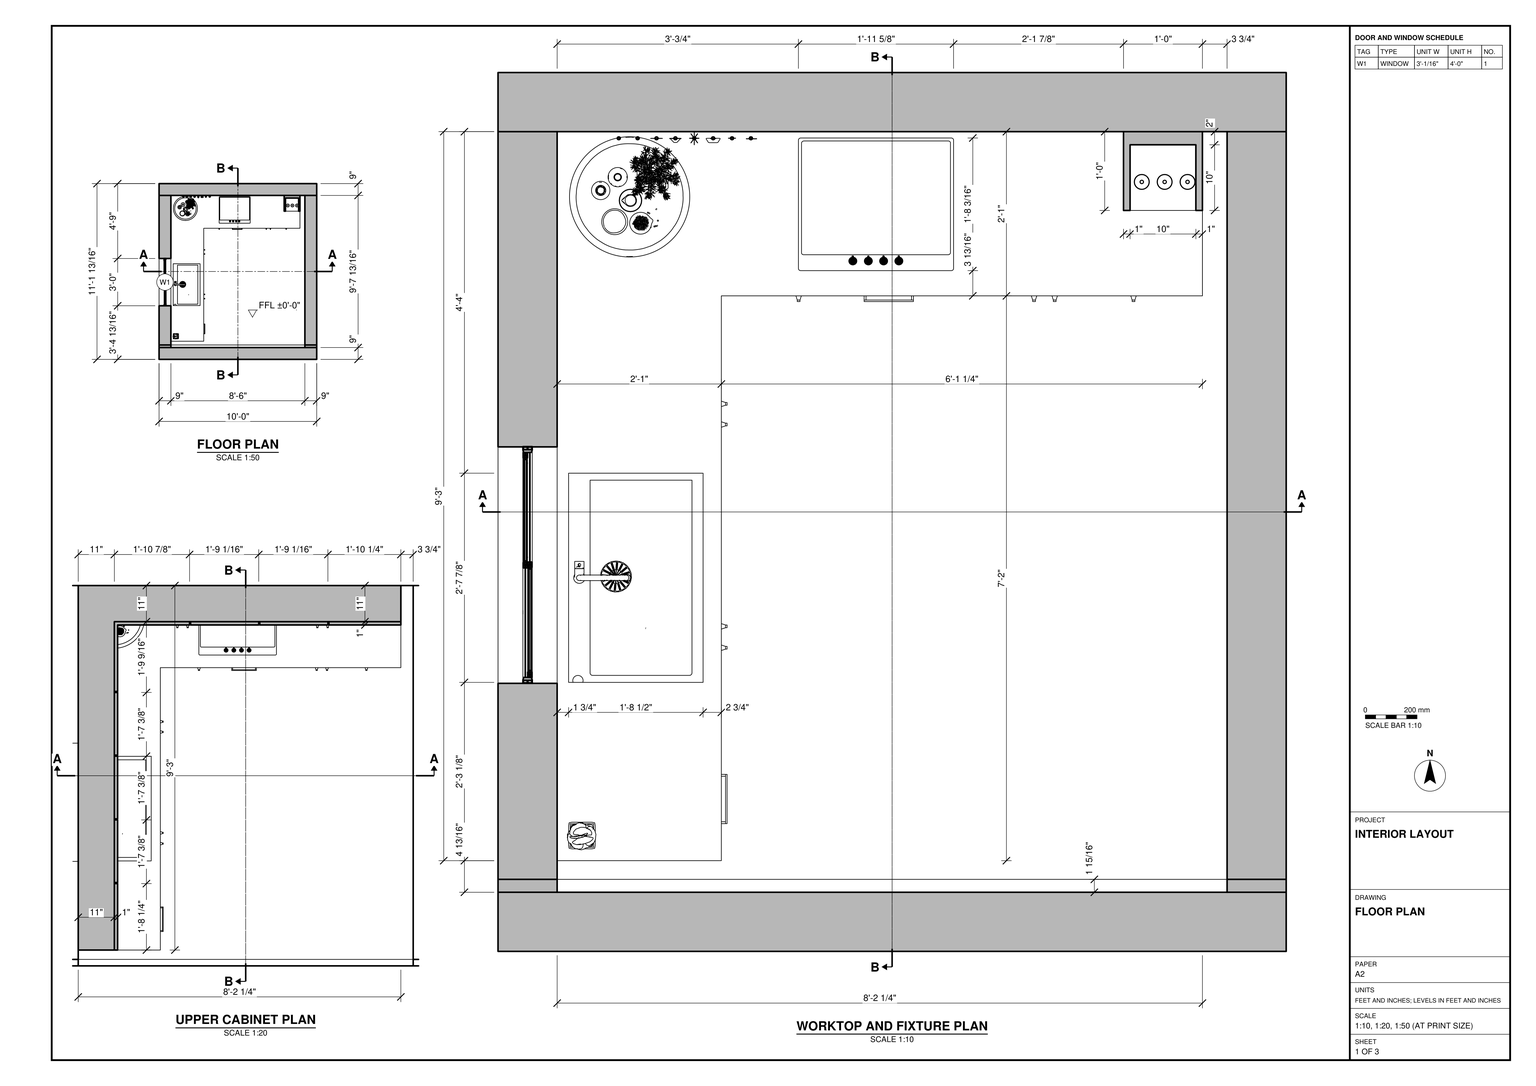
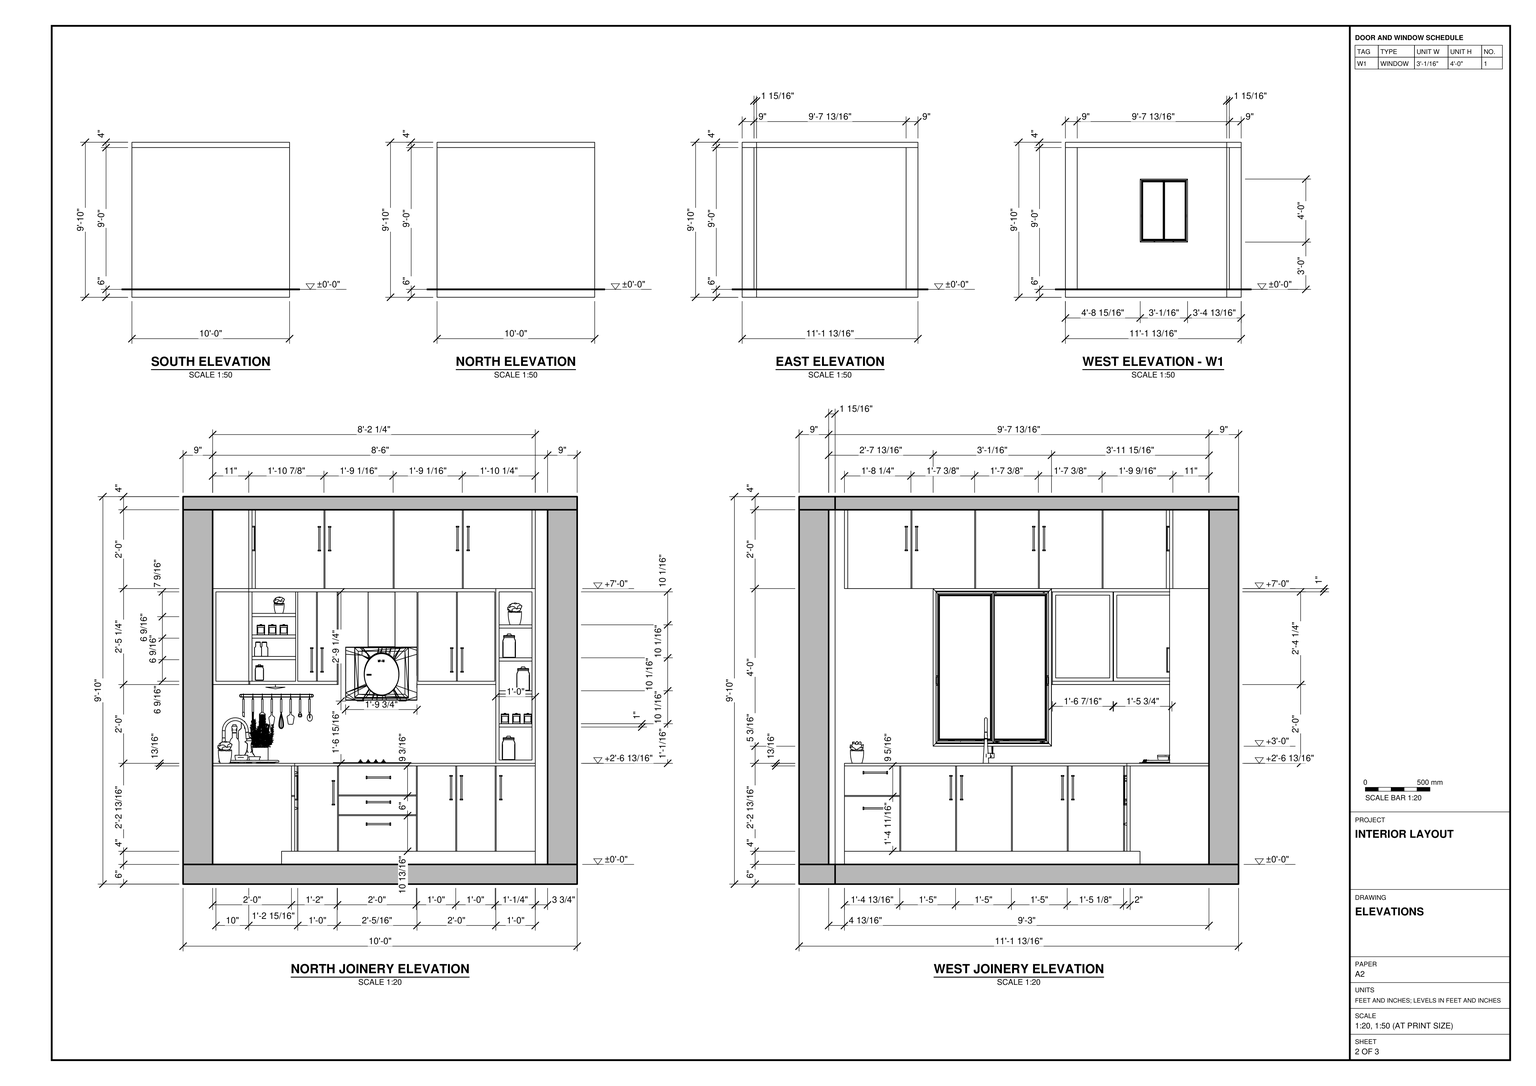
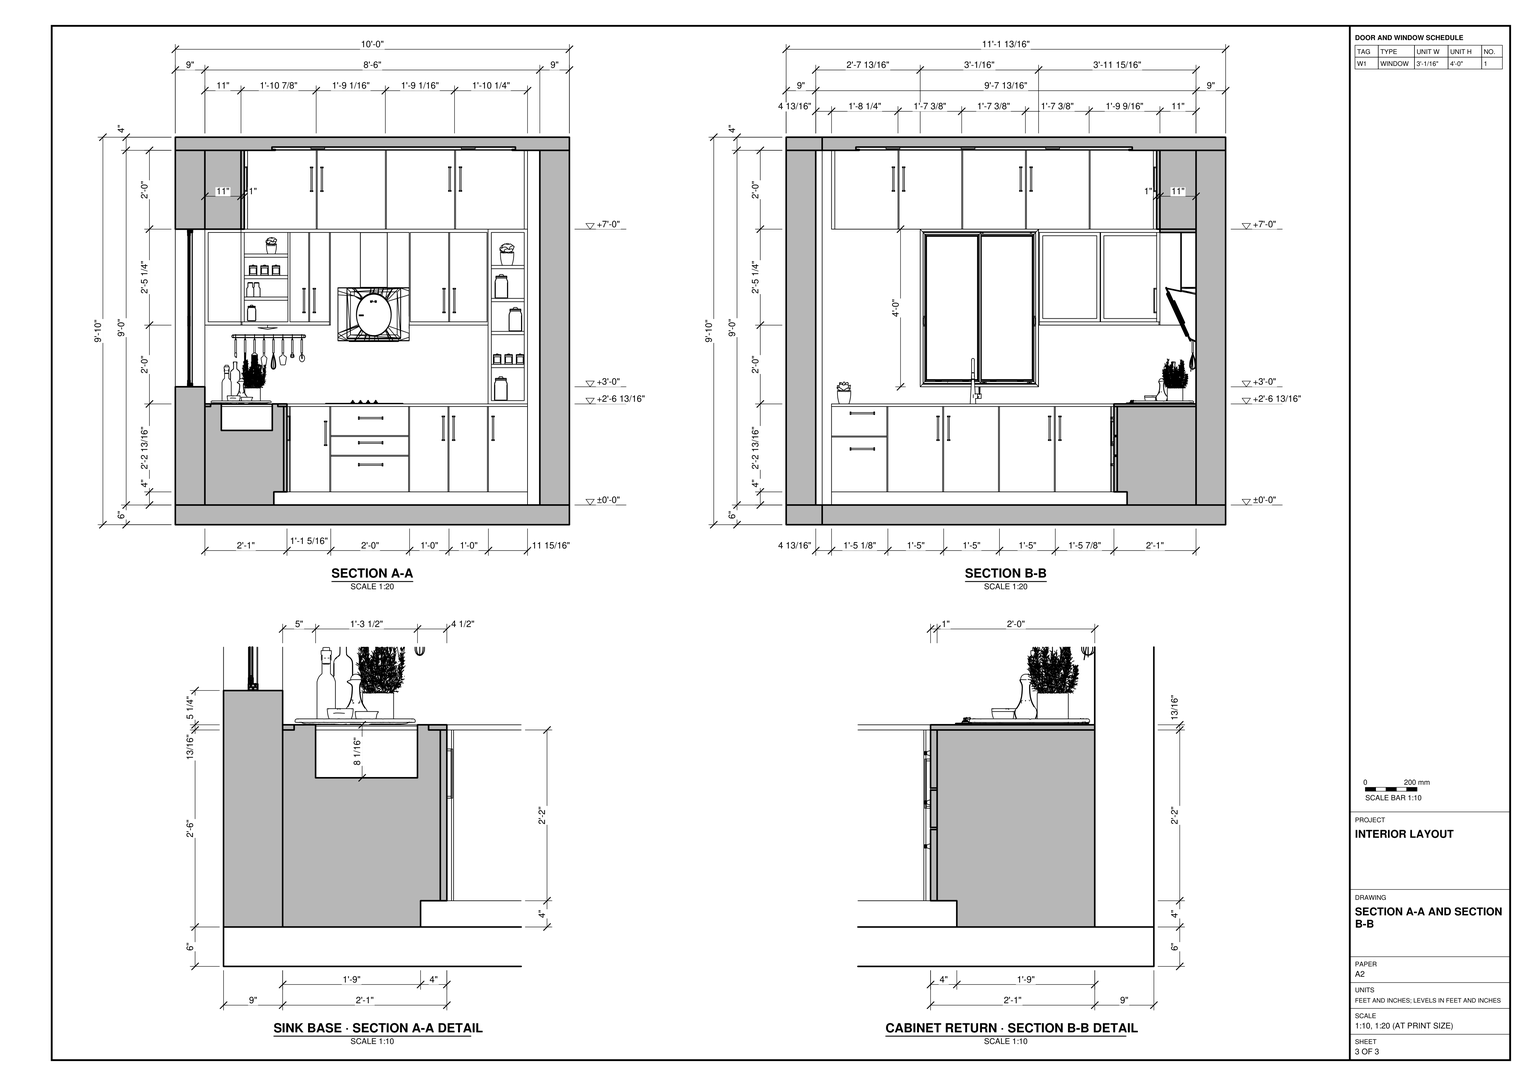
Build the kitchen in SketchUp from task_files/diagram_01.pdf. Work in feet and inches. Set the finished floor at ±0'-0". The room shell measures 10'-0" east to west by 11'-1 13/16" north to south, with an overall height of 9'-10". Model the 9" perimeter walls between the 6" floor slab and the 4" top slab. Fit the two-panel window in the west wall, with its sill above the sink as shown in the section.

Use the worktop plan to lay out the continuous L-shaped counter, with the sink and faucet on the west run and the cooktop on the north run. Follow the joinery elevations for the base cupboards, drawer stacks, handles, open shelves and upper cabinets. Align the extractor hood with the cooktop and the drawers below it. Use the enlarged sections to set the basin into the worktop and recess the plinths behind the cabinet fronts. Keep the upper cabinets clear of the window opening.

Decor, appliances and loose items such as jars, utensils and plants may be any suitable library components placed as shown. Keep shell elements and individual furniture or joinery pieces in separate groups or components, and use components for repeated parts. Save one SketchUp model as output_files/kitchen_with_l_shaped_cabinetry_and_a_west_window.skp.

# SketchUp Ruby script. Lengths in inches.
U = 1.inch
M = Sketchup.active_model
def pt(a) = Geom::Point3d.new(a.map { |v| v * U })
def face(e, loops, mat)
  f = e.add_face(loops[0].map { |a| pt(a) })
  loops[1..].each { |l| e.add_face(l.map { |a| pt(a) }).erase! }
  f.material = f.back_material = mat if mat
  f
end
# faces: each face lists its corners as indices into pts; further lists are holes
def faces(e, pts, list, mat = nil) = list.each { |f| face(e, (f[0].is_a?(Array) ? f : [f]).map { |l| l.map { |i| pts[i] } }, mat) }
# xy, xz, yz: faces in a plane at the given z, y or x. An outline is a flat list of corners, or four numbers for a rectangle; further outlines are holes
def ring(l) = l.size == 4 ? [[l[0], l[1]], [l[2], l[1]], [l[2], l[3]], [l[0], l[3]]] : l.each_slice(2).to_a
def flat(e, list, mat, &to3) = list.each { |f| face(e, (f[0].is_a?(Array) ? f : [f]).map { |l| ring(l).map { |u, v| to3.(u, v) } }, mat) }
def xy(e, z, list, mat = nil) = flat(e, list, mat) { |x, y| [x, y, z] }
def xz(e, y, list, mat = nil) = flat(e, list, mat) { |x, z| [x, y, z] }
def yz(e, x, list, mat = nil) = flat(e, list, mat) { |y, z| [x, y, z] }
def lines(e, pts, list) = list.each { |a, b| e.add_line(pt(pts[a]), pt(pts[b])) }
# prism: a flat outline (further loops are holes) pulled along v
def prism(e, loops, v, mat = nil)
  f = face(e, loops, mat); d = Geom::Vector3d.new(v.map { |x| x * U })
  f.pushpull(f.normal.samedirection?(d) ? d.length : -d.length)
end
def box(e, o, s, mat = nil) = prism(e, [[o, [o[0] + s[0], o[1], o[2]], [o[0] + s[0], o[1] + s[1], o[2]], [o[0], o[1] + s[1], o[2]]]], [0, 0, s[2]], mat)
def at(x, y, z, deg = 0) = Geom::Transformation.translation(pt([x, y, z])) * Geom::Transformation.rotation(ORIGIN, Z_AXIS, deg.degrees)
def axes(o, x, y, z) = Geom::Transformation.new([*x, 0, *y, 0, *z, 0, *pt(o).to_a, 1])
def part(name) = M.definitions.add(name)
# library, detail: a bought-in or finely detailed component or shape, given as its bounding box
def library(name, o, s) = part(name).tap { |d| box(d.entities, o, s) }
def detail(e, o, s) = box(e.add_group.entities, o, s)
def put(e, d, t, mat = nil) = e.add_instance(d, t).tap { |i| i.material = mat if mat }
def group(e, t, mat = nil) = e.add_group.tap { |g| g.transformation = t; g.material = mat if mat }.entities
root = M.entities
M.materials.add("Emissive").color = [255, 242, 225]
M.materials["Emissive"].alpha = 1
M.materials.add("Manhattan Creative Coating ML 1016B 24.75cm").color = [255, 255, 255]
M.materials.add("Marble Beige 23-86 150cm").color = [204, 192, 177]
M.materials.add("Marble Black 01 150cm").color = [31, 31, 31]
M.materials.add("Wood Mahogany 33-46 100cm\#2").color = [84, 42, 21]
M.materials.add("Wood Teak 33-35 100cm").color = [135, 81, 33]
M.materials.add("[Color M09]").color = [0, 0, 0]
M.materials.add("[Translucent Glass Blue]").color = [100, 149, 237]
M.materials["[Translucent Glass Blue]"].alpha = 0.5
c1 = library("Window Crafter Sliding",[0,-0.1,0],[78.74,3.59,94.49])
c2 = part("Square panel")
box(c2.entities,[0,0,0],[10.02,10,1],"Wood Mahogany 33-46 100cm\#2")
c3 = part("Component\#4")
box(c3.entities,[0,1,0],[13.97,9,1])
c4 = part("Component\#6")
box(c4.entities,[0,0,0],[9,18.46,1])
c5 = part("Component\#7")
box(c5.entities,[0,0,0],[9,17.75,1])
c6 = library("sink",[-18.39,0,-10.63],[31.85,20.47,24.5])
c7 = library("Chimney",[0,-14.34,0],[33.95,14.34,33.72])
c8 = part("POI-E1497-320-1917\#1")
xy(c8.entities,0,[[0,0,0.29,0.83],[7.21,0,7.5,0.83]])
xy(c8.entities,0.64,[[0.29,0.21,7.21,0.62]])
xy(c8.entities,0.875,[[0,0.21,7.5,0.62]])
xz(c8.entities,0.21,[[0,0.64,7.5,0.875]])
xz(c8.entities,0.62,[[0,0.64,7.5,0.875]])
yz(c8.entities,0,[[0,0,0.21,0.64,0.21,0.875,0.62,0.875,0.62,0.64,0.83,0]])
yz(c8.entities,0.29,[[0,0,0.83,0,0.62,0.64,0.21,0.64]])
yz(c8.entities,7.21,[[0,0,0.21,0.64,0.62,0.64,0.83,0]])
yz(c8.entities,7.5,[[0,0,0.83,0,0.62,0.64,0.62,0.875,0.21,0.875,0.21,0.64]])
p = [[0,0.21,0.64],[0,0,0],[0.29,0,0],[0.29,0.21,0.64],[7.21,0.21,0.64],[7.21,0,0],
  [7.5,0,0],[7.5,0.21,0.64],[0,0.83,0],[0,0.62,0.64],[0.29,0.62,0.64],[0.29,0.83,0],
  [7.5,0.83,0],[7.5,0.62,0.64],[7.21,0.62,0.64],[7.21,0.83,0]]
faces(c8.entities,p,[[0,1,2,3],[4,5,6,7],[8,9,10,11],[12,13,14,15]])
c9 = library("1045",[78.33,40.52,-0.08],[23.62,20.2,1.2])
c10 = library("kitchen",[57.57,5.21,10.61],[18.31,18.31,13.72])
c11 = library("Kitchen Utensils 20-56",[-15.41,-1.59,-10.72],[30.82,2.02,11.3])
c12 = library("Glass Vessel 001",[-1.95,-1.95,0.02],[3.9,3.9,7.26])
c13 = library("Kitchen Utensils Jugs 92-07",[-4.45,-3.74,0],[8.9,7.5,9.62])
c14 = library("jars",[-1.97,-1.97,0],[15.75,3.94,5.39])
c15 = library("Potted Plant 50-24",[-2.18,-2.1,0],[4.36,4.2,6.7])
c16 = part("Group319\#1")
p = [[0,0,0],[0,0,-1.83],[-0.77,0,-1.83],[5.01,-0.92,0],[-5.01,-0.92,0],[5.01,0.92,0],
  [5.01,0,0],[-5.01,0.92,0],[0.77,0,-1.83],[-5.01,0,0],[0,0,-2.96]]
lines(c16.entities,p,[[0,1],[1,2],[3,4],[5,6],[7,5],[1,8],[9,0],[0,6],[8,10],[4,9],[6,3],[2,10],
  [9,7]])
c17 = part("Rectangle Light")
put(c17.entities,c16,at(0,0,0))
c18 = part("Group321\#1")
p = [[0,0,0],[0,0,-1.81],[-0.77,0,-1.81],[5.01,-0.84,0],[-5.01,-0.84,0],[5.01,0.84,0],
  [5.01,0,0],[-5.01,0.84,0],[0.77,0,-1.81],[-5.01,0,0],[0,0,-2.93]]
lines(c18.entities,p,[[0,1],[1,2],[3,4],[5,6],[7,5],[1,8],[9,0],[0,6],[8,10],[4,9],[6,3],[2,10],
  [9,7]])
c19 = part("Rectangle Light\#1")
put(c19.entities,c18,at(0,0,0))
c20 = part("Group323\#1")
p = [[0,0,0],[0,0,-2],[-0.77,0,-2],[5.01,-1.47,0],[-5.01,-1.47,0],[5.01,1.47,0],
  [5.01,0,0],[-5.01,1.47,0],[0.77,0,-2],[-5.01,0,0],[0,0,-3.24]]
lines(c20.entities,p,[[0,1],[1,2],[3,4],[5,6],[7,5],[1,8],[9,0],[0,6],[8,10],[4,9],[6,3],[2,10],
  [9,7]])
c21 = part("Rectangle Light\#2")
put(c21.entities,c20,at(0,0,0))
c22 = part("Group325\#3")
p = [[0,0,0],[0,0,-1.85],[-0.77,0,-1.85],[5.01,-0.98,0],[-5.01,-0.98,0],[5.01,0.98,0],
  [5.01,0,0],[-5.01,0.98,0],[0.77,0,-1.85],[-5.01,0,0],[0,0,-2.99]]
lines(c22.entities,p,[[0,1],[1,2],[3,4],[5,6],[7,5],[1,8],[9,0],[0,6],[8,10],[4,9],[6,3],[2,10],
  [9,7]])
c23 = part("Rectangle Light\#3")
put(c23.entities,c22,at(0,0,0))
c24 = part("Group327\#1")
p = [[0,0,0],[0,0,-1.97],[-0.77,0,-1.97],[5.01,-1.38,0],[-5.01,-1.38,0],[5.01,1.38,0],
  [5.01,0,0],[-5.01,1.38,0],[0.77,0,-1.97],[-5.01,0,0],[0,0,-3.19]]
lines(c24.entities,p,[[0,1],[1,2],[3,4],[5,6],[7,5],[1,8],[9,0],[0,6],[8,10],[4,9],[6,3],[2,10],
  [9,7]])
c25 = part("Rectangle Light\#4")
put(c25.entities,c24,at(0,0,0))
c26 = part("Group329\#1")
p = [[0,0,0],[0,0,-2.64],[-1.07,0,-2.64],[6.99,-1.58,0],[-6.99,-1.58,0],[6.99,1.58,0],
  [6.99,0,0],[-6.99,1.58,0],[1.07,0,-2.64],[-6.99,0,0],[0,0,-4.28]]
lines(c26.entities,p,[[0,1],[1,2],[3,4],[5,6],[7,5],[1,8],[9,0],[0,6],[8,10],[4,9],[6,3],[2,10],
  [9,7]])
c27 = part("Rectangle Light\#5")
put(c27.entities,c26,at(0,0,0))
c28 = part("Group331\#1")
p = [[0,0,0],[0,0,-2.47],[-1.07,0,-2.47],[6.99,-1.01,0],[-6.99,-1.01,0],[6.99,1.01,0],
  [6.99,0,0],[-6.99,1.01,0],[1.07,0,-2.47],[-6.99,0,0],[0,0,-4]]
lines(c28.entities,p,[[0,1],[1,2],[3,4],[5,6],[7,5],[1,8],[9,0],[0,6],[8,10],[4,9],[6,3],[2,10],
  [9,7]])
c29 = part("Rectangle Light\#6")
put(c29.entities,c28,at(0,0,0))
c30 = part("Group333\#1")
p = [[0,0,0],[0,0,-2.5],[-1.07,0,-2.5],[6.99,-1.09,0],[-6.99,-1.09,0],[6.99,1.09,0],
  [6.99,0,0],[-6.99,1.09,0],[1.07,0,-2.5],[-6.99,0,0],[0,0,-4.04]]
lines(c30.entities,p,[[0,1],[1,2],[3,4],[5,6],[7,5],[1,8],[9,0],[0,6],[8,10],[4,9],[6,3],[2,10],
  [9,7]])
c31 = part("Rectangle Light\#7")
put(c31.entities,c30,at(0,0,0))
c32 = part("Group335\#1")
p = [[0,0,0],[0,0,-2.52],[-1.07,0,-2.52],[6.99,-1.16,0],[-6.99,-1.16,0],[6.99,1.16,0],
  [6.99,0,0],[-6.99,1.16,0],[1.07,0,-2.52],[-6.99,0,0],[0,0,-4.07]]
lines(c32.entities,p,[[0,1],[1,2],[3,4],[5,6],[7,5],[1,8],[9,0],[0,6],[8,10],[4,9],[6,3],[2,10],
  [9,7]])
c33 = part("Rectangle Light\#8")
put(c33.entities,c32,at(0,0,0))
c34 = library("Tlon Light 650 Ceiling 152 007",[-12.8,-12.8,-3.78],[25.6,25.6,3.58])
c35 = part("Group347\#3")
p = [[0,0,0],[0,0,-4.23],[-1.84,0,-4.23],[12,-1.68,0],[-12,-1.68,0],[12,1.68,0],
  [12,0,0],[-12,1.68,0],[1.84,0,-4.23],[-12,0,0],[0,0,-6.84]]
lines(c35.entities,p,[[0,1],[1,2],[3,4],[5,6],[7,5],[1,8],[9,0],[0,6],[8,10],[4,9],[6,3],[2,10],
  [9,7]])
c36 = part("Rectangle Light\#10")
put(c36.entities,c35,at(0,0,0))
c37 = library("Group\#23",[-0.04,-0.04,0],[3.03,9.65,3.68])
c38 = part("Group345\#1")
p = [[0,0,0],[0,0,-6.68],[-2.9375,0,-6.68],[19.12,-2.51,0],[-19.12,-2.51,0],[19.12,2.51,0],
  [19.12,0,0],[-19.12,2.51,0],[2.9375,0,-6.68],[-19.12,0,0],[0,0,-10.8125]]
lines(c38.entities,p,[[0,1],[1,2],[3,4],[5,6],[7,5],[1,8],[9,0],[0,6],[8,10],[4,9],[6,3],[2,10],
  [9,7]])
c39 = part("Rectangle Light\#9")
put(c39.entities,c38,at(0,0,0))
c40 = part("Group343\#1")
xz(c40.entities,22.6,[[26.53,0,146.53,6]])
c41 = part("Group347\#1")
xz(c41.entities,22.6,[[26.53,6,35.53,114]])
c42 = part("Group1235\#1")
xz(c42.entities,22.6,[[137.53,6,146.53,114]])
c43 = part("Group1237\#1")
xz(c43.entities,22.6,[[26.53,114,146.53,118]])
c44 = part("Group340\#3")
put(c44.entities,c40,at(0,0,0))
put(c44.entities,c41,at(0,0,0))
put(c44.entities,c42,at(0,0,0))
put(c44.entities,c43,at(0,0,0))
box(root,[0,0,6],[120,9,108])
p = [[71.02,100.8125,10],[47.34,100.8125,10],[71.02,100.8125,20.84],[71.02,100.8125,26.84],[47.34,100.8125,26.84],[47.34,100.8125,21.16],
  [71.02,100.8125,21.16],[47.34,100.8125,20.84],[29.1875,42.02,36],[29.24,42.03,36],[29.29,42.05,36],[29.33,42.07,36],
  [14.26,42.05,36],[14.31,42.03,36],[14.07,42.22,36],[14.1,42.17,36],[29.5,42.26,36],[29.52,42.3125,36],
  [14.03,42.3125,36],[14.04,42.26,36],[14.02,42.42,36],[14.02,42.36,36],[14.17,42.1,36],[14.21,42.07,36],
  [14.13,42.13,36],[14.36,42.02,36],[14.41,42.02,36],[29.53,71.75,36],[14.02,71.75,36],[29.13,42.02,36],
  [29.41,42.13,36],[29.45,42.17,36],[29.375,42.1,36],[29.48,42.22,36],[29.52,42.36,36],[12.16,56.0625,36.79],
  [12.38,56.03,36.79],[11.95,56.15,36.79],[11.76,56.28,36.79],[11.625,56.46,36.79],[11.54,56.66,36.79],[11.51,56.88,36.79],
  [11.54,57.1,36.79],[11.625,57.3,36.79],[11.76,57.48,36.79],[11.95,57.61,36.79],[12.16,57.7,36.79],[12.38,57.73,36.79],
  [12.61,57.7,36.79],[12.82,57.61,36.79],[13,57.48,36.79],[13.14,57.3,36.79],[13.22,57.1,36.79],[13.25,56.88,36.79],
  [13.22,56.66,36.79],[13.14,56.46,36.79],[13,56.28,36.79],[12.82,56.15,36.79],[12.61,56.0625,36.79],[33,47.65,10],
  [33,47.65,36],[71.02,100.8125,27.16],[71.02,100.8125,36],[33,100.8125,10],[47.02,100.8125,10],[107.25,100.8125,10],
  [107.25,100.8125,36],[95.02,100.8125,10],[83.34,100.8125,10],[33,100.8125,36],[33,64.64,10],[33,64.96,10],
  [33,47.96,10],[95.34,100.8125,10],[33,30.97,36],[33,30.97,10],[33,13.8125,27],[33,13.8125,36],
  [95.02,100.8125,36],[47.34,100.8125,27.16],[71.34,100.8125,36],[71.34,100.8125,10],[83.02,100.8125,10],[83.02,100.8125,36],
  [33,81.64,10],[33,81.64,36],[33,30.65,27],[83.34,100.8125,36],[95.23,124.8125,36.79],[95.23,112.8125,36.79],
  [107.25,112.8125,36.79],[33,13.8125,26.69],[33,13.8125,10],[33,81.95,10],[33,81.95,36],[33,30.65,26.69],
  [33,30.65,10],[47.02,100.8125,36],[33,64.64,36],[33,30.65,36],[33,47.96,36],[33,64.96,36],
  [47.34,100.8125,36],[107.25,124.8125,36.79],[95.34,100.8125,36],[107.25,124.8125,6],[107.25,103.8125,6],[9,124.8125,6],
  [9,13.8125,6],[30,13.8125,6],[30,103.8125,6],[9,13.8125,36],[9,13.8125,36.79],[9,124.8125,36],
  [107.25,124.8125,36],[9,124.8125,36.79]]
lines(root,p,[[0,1],[0,2],[3,4],[4,5],[5,6],[2,7],[7,1],[6,3],[8,9],[10,11],[12,13],[14,15],
  [16,17],[18,19],[20,21],[22,23],[24,22],[13,25],[25,26],[27,28],[26,29],[23,12],[9,10],[30,31],
  [21,18],[11,32],[31,33],[15,24],[33,16],[32,30],[19,14],[29,8],[17,34],[34,27],[28,20],[35,36],
  [37,35],[38,37],[39,38],[40,39],[41,40],[42,41],[43,42],[44,43],[45,44],[46,45],[47,46],[48,47],
  [49,48],[50,49],[51,50],[52,51],[53,52],[54,53],[55,54],[56,55],[57,56],[58,57],[36,58],[59,60],
  [61,62],[63,64],[65,66],[67,68],[69,63],[70,71],[59,72],[65,73],[74,75],[76,77],[67,78],[79,61],
  [80,81],[72,70],[82,83],[84,85],[76,86],[75,59],[87,68],[88,89],[89,90],[91,92],[84,93],[94,93],
  [95,91],[92,96],[64,97],[70,98],[96,95],[71,84],[86,99],[100,72],[101,71],[102,79],[90,103],[96,75],
  [93,63],[82,81],[104,73],[105,106],[105,107],[107,108],[109,110],[106,110],[74,60],[77,99],[111,77],[111,112],
  [113,111],[114,66],[114,103],[114,113],[103,88],[113,115],[69,97],[108,111],[107,113],[105,114],[115,112],[100,98],
  [85,94],[104,66],[78,104],[80,83],[97,102],[88,115],[101,85],[87,78],[62,80],[60,100],[62,102],[99,74],
  [83,87],[94,69],[98,101],[109,108]])
put(root,c1,axes([3.79,76.86,42],[0,-0.4578,0],[0.42,0,0],[0,0,0.508]))
put(root,c2,at(96.23,112.8125,47.83))
put(root,c2,at(96.23,112.8125,57.87))
put(root,c2,at(96.23,112.8125,67.91))
put(root,c2,at(96.23,112.8125,77.96),"Wood Mahogany 33-46 100cm\#2")
put(root,c3,at(20.31,113.8125,68.34))
put(root,c3,at(20.31,113.8125,74.89))
put(root,c3,at(20.31,113.8125,81.45))
put(root,c4,at(10,77.13,70.52))
put(root,c4,at(10,77.13,79.26))
put(root,c5,at(10,95.75,70.52))
put(root,c5,at(10,95.75,79.26))
put(root,c6,at(31.22,59.34,36.79,90))
put(root,c7,axes([49.5,124.8125,54.79],[0.64,0,0],[0,0.64,0],[0,0,1.01456]))
put(root,c8,axes([34,26.95,34.36],[0,-1,0],[0,0,-1],[1,0,0]))
put(root,c8,axes([34,26.95,23.48],[0,-1,0],[0,0,-1],[1,0,0]))
put(root,c8,axes([63.24,99.8125,32.88],[-1,0,0],[0,0,-1],[0,-1,0]))
put(root,c8,axes([34,45.82,33.11],[0,0,-1],[0,1,0],[1,0,0]))
put(root,c8,axes([34,79.81,33.11],[0,0,-1],[0,1,0],[1,0,0]))
put(root,c8,axes([34,49.08,33.11],[0,0,-1],[0,1,0],[1,0,0]))
put(root,c8,axes([34,82.95,33.11],[0,0,-1],[0,1,0],[1,0,0]))
put(root,c8,axes([63.24,99.8125,25.38],[-1,0,0],[0,0,-1],[0,-1,0]))
put(root,c8,axes([63.24,99.8125,18.69],[-1,0,0],[0,0,-1],[0,-1,0]))
put(root,c8,axes([45.35,99.8125,31.57],[0,0,-1],[1,0,0],[0,-1,0]))
put(root,c8,axes([96.34,99.8125,33.11],[0,0,-1],[1,0,0],[0,-1,0]))
put(root,c8,axes([84.34,99.8125,33.11],[0,0,-1],[1,0,0],[0,-1,0]))
put(root,c8,axes([81.19,99.8125,33.11],[0,0,-1],[1,0,0],[0,-1,0]))
put(root,c8,axes([41.07,112.8125,108.9375],[0,0,-1],[1,0,0],[0,-1,0]))
put(root,c8,axes([44.22,112.8125,108.9375],[0,0,-1],[1,0,0],[0,-1,0]))
put(root,c8,axes([86.41,112.8125,109],[0,0,-1],[1,0,0],[0,-1,0]))
put(root,c8,axes([83.16,112.8125,109],[0,0,-1],[1,0,0],[0,-1,0]))
put(root,c8,axes([21,32.23,109],[0,0,-1],[0,1,0],[1,0,0]))
put(root,c8,axes([21,71.03,109],[0,0,-1],[0,1,0],[1,0,0]))
put(root,c8,axes([21,74.17,109],[0,0,-1],[0,1,0],[1,0,0]))
put(root,c8,axes([21,35.37,109],[0,0,-1],[0,1,0],[1,0,0]))
put(root,c9,at(-32.59,63.125,36.87))
put(root,c10,at(-46.6875,100.52,26.18))
put(root,c11,axes([28.44,124.39,57.38],[0.73,0,0],[0,1,0],[0,0,1]))
put(root,c12,at(99.13,118.67,37.79))
put(root,c12,at(99.29,118.16,68.91))
put(root,c12,at(103.55,117.7,58.87))
put(root,c12,axes([23.24,118.63,62.05],[0.66,0,0],[0,0.66,0],[0,0,0.66]))
put(root,c13,axes([23.78,121.08,69.34],[0.46,0,0],[0,0.46,0],[0,0,0.46]))
put(root,c13,axes([12.05,81.45,71.52],[0.46,0,0],[0,0.46,0],[0,0,0.46]))
put(root,c12,axes([14.1,80.99,61.77],[0.66,0,0],[0,0.66,0],[0,0,0.66]))
put(root,c12,axes([14.1,97.67,61.77],[0.66,0,0],[0,0.66,0],[0,0,0.66]))
put(root,c12,axes([14.1,97.67,80.15],[0.66,0,0],[0,0.66,0],[0,0,0.66]))
put(root,c13,axes([12.05,88.08,71.52],[0.46,0,0],[0,0.46,0],[0,0,0.46]))
put(root,c12,axes([12.36,104.19,80.25],[0.66,0,0],[0,0.66,0],[0,0,0.66]))
put(root,c14,axes([23.69,116.9,75.89],[0.59,0,0],[0,0.59,0],[0,0,0.59]))
put(root,c14,axes([98.01,117.16,48.83],[0.59,0,0],[0,0.59,0],[0,0,0.59]))
put(root,c15,at(100.98,115.6875,78.96))
put(root,c15,axes([29.22,118.1875,82.45],[0.75,0,0],[0,0.75,0],[0,0,0.75]))
put(root,c15,at(15.67,109.55,61.79))
put(root,c15,at(12.72,17.56,36.79))
put(root,c8,axes([38.77,112.8125,72.01],[0,0,-1],[1,0,0],[0,-1,0]))
put(root,c8,axes([41.92,112.8125,72.01],[0,0,-1],[1,0,0],[0,-1,0]))
put(root,c8,axes([84.55,112.8125,72.01],[0,0,-1],[1,0,0],[0,-1,0]))
put(root,c8,axes([81.4,112.8125,72.01],[0,0,-1],[1,0,0],[0,-1,0]))
put(root,c17,axes([101.24,121.89,88.99],[1,0,0],[0,-1,0],[0,0,0.27]))
put(root,c19,axes([101.24,121.97,77.95],[1,0,0],[0,-1,0],[0,0,0.18]))
put(root,c21,axes([101.24,121.35,67.9],[1,0,0],[0,-1,0],[0,0,0.31]))
put(root,c23,axes([101.24,121.83,57.86],[1,0,0],[0,-1,0],[0,0,0.11]))
put(root,c25,axes([101.24,121.43,47.82],[1,0,0],[0,-1,0],[0,0,0.15]))
put(root,c27,axes([27.3,122.24,88.99],[1,0,0],[0,-1,0],[0,0,0.17]))
put(root,c29,axes([27.3,122.8,81.4375],[1,0,0],[0,-1,0],[0,0,0.19]))
put(root,c31,axes([27.3,122.72,74.88],[1,0,0],[0,-1,0],[0,0,0.21]))
put(root,c33,axes([27.3,122.65,68.33],[1,0,0],[0,-1,0],[0,0,0.18]))
put(root,c34,axes([43.39,81.13,115],[0.16498,0,0],[0,0.16498,0],[0,0,0.16498]))
put(root,c34,axes([89.2,81.13,115],[0.16498,0,0],[0,0.16498,0],[0,0,0.16498]))
put(root,c34,axes([89.2,55.38,115],[0.16498,0,0],[0,0.16498,0],[0,0,0.16498]))
put(root,c34,axes([43.39,55.38,115],[0.16498,0,0],[0,0.16498,0],[0,0,0.16498]))
put(root,c34,axes([89.2,32.51,115],[0.16498,0,0],[0,0.16498,0],[0,0,0.16498]))
put(root,c34,axes([43.39,32.51,115],[0.16498,0,0],[0,0.16498,0],[0,0,0.16498]))
put(root,c36,axes([83.23,123.13,60.78],[1,0,0],[0,-1,0],[0,0,0.22]))
g1 = group(root,at(0,13.8125,0))
xy(g1,0,[[0,-13.8125,120,120]])
xy(g1,6,[[0,-13.8125,120,120]],"Marble Beige 23-86 150cm")
xz(g1,-13.8125,[[0,0,120,6]])
xz(g1,120,[[0,0,120,6]])
yz(g1,0,[[-13.8125,0,120,6]])
yz(g1,120,[[-13.8125,0,120,6]])
g2 = group(root,at(0,124.8125,6))
xy(g2,0,[[0,0,120,9]])
xy(g2,108,[[0,0,120,9]])
xz(g2,0,[[0,0,120,108]],"Marble Beige 23-86 150cm")
xz(g2,9,[[0,0,120,108]])
yz(g2,0,[[0,0,9,108]])
yz(g2,120,[[0,0,9,108]])
g3 = group(root,at(0,13.8125,6))
xy(g3,0,[[0,-4.8125,9,111]])
xy(g3,36,[[0,27,9,63]])
xy(g3,84,[[0,27,9,63]])
xy(g3,108,[[0,-4.8125,9,111]])
xz(g3,-4.8125,[[0,0,9,108]])
xz(g3,27,[[0,36,9,84]])
xz(g3,63,[[0,36,9,84]])
xz(g3,111,[[0,0,9,108]])
yz(g3,0,[[[-4.8125,0,111,108],[27,36,63,84]]])
yz(g3,9,[[[-4.8125,0,111,108],[27,36,63,84]]],"Marble Beige 23-86 150cm")
g4 = group(root,at(33,13.8125,10),"Manhattan Creative Coating ML 1016B 24.75cm")
xy(g4,0,[[0,0,1,16.84],[0,17.15,1,33.83],[0,34.15,1,50.83],[0,51.14,1,67.82],[0,68.14,0,87,14.02,87,14.02,86,1,86,1,68.14],
  [14.34,86,38.02,87],[38.34,86,50.02,87],[50.34,86,62.02,87],[62.34,86,74.25,87]])
xy(g4,10.84,[[14.34,86,38.02,87]])
xy(g4,11.16,[[14.34,86,38.02,87]])
xy(g4,16.69,[[0,0,1,16.84]])
xy(g4,16.84,[[14.34,86,38.02,87]])
xy(g4,17,[[0,0,1,16.84]])
xy(g4,17.16,[[14.34,86,38.02,87]])
xy(g4,26,[[0,0,1,16.84],[0,17.15,1,33.83],[0,34.15,1,50.83],[0,51.14,1,67.82],[0,68.14,1,68.14,1,86,14.02,86,14.02,87,0,87],
  [14.34,86,38.02,87],[38.34,86,50.02,87],[50.34,86,62.02,87],[62.34,86,74.25,87]])
xz(g4,0,[[0,0,1,16.69],[0,17,1,26]])
xz(g4,16.84,[[0,0,1,16.69],[0,17,1,26]])
xz(g4,17.15,[[0,0,1,26]])
xz(g4,33.83,[[0,0,1,26]])
xz(g4,34.15,[[0,0,1,26]])
xz(g4,50.83,[[0,0,1,26]])
xz(g4,51.14,[[0,0,1,26]])
xz(g4,67.82,[[0,0,1,26]])
xz(g4,68.14,[[0,0,1,26]])
xz(g4,86,[[1,0,1.71,26],[1.71,0,2.02,26],[2.02,0,14.02,26],[14.34,0,38.02,10.84],[38.34,0,50.02,26],
  [50.34,0,62.02,26],[62.34,0,74.25,26],[14.34,11.16,38.02,16.84],[14.34,17.16,38.02,26]])
xz(g4,87,[[0,0,14.02,26],[14.02,0,14.34,26],[14.34,0,38.02,10.84],[38.02,0,38.34,26],[38.34,0,50.02,26],
  [50.02,0,50.34,26],[50.34,0,62.02,26],[62.02,0,62.34,26],[62.34,0,74.25,26],[14.34,10.84,38.02,11.16],
  [14.34,11.16,38.02,16.84],[14.34,16.84,38.02,17.16],[14.34,17.16,38.02,26]])
yz(g4,0,[[0,0,16.84,16.69],[16.84,0,17.15,26],[17.15,0,33.83,26],[33.83,0,34.15,26],[34.15,0,50.83,26],
  [50.83,0,51.14,26],[51.14,0,67.82,26],[67.82,0,68.14,26],[68.14,0,87,26],[0,16.69,16.84,17],
  [0,17,16.84,26]])
yz(g4,1,[[0,0,16.84,16.69],[17.15,0,33.83,26],[34.15,0,50.83,26],[51.14,0,67.82,26],[68.14,0,84.98,26],
  [84.98,0,85.29,26],[85.29,0,86,26]])
yz(g4,1,[[0,17,16.84,26]],"Manhattan Creative Coating ML 1016B 24.75cm")
yz(g4,14.02,[[86,0,87,26]])
yz(g4,14.34,[[86,0,87,10.84],[86,11.16,87,16.84],[86,17.16,87,26]])
yz(g4,38.02,[[86,0,87,10.84],[86,11.16,87,16.84],[86,17.16,87,26]])
yz(g4,38.34,[[86,0,87,26]])
yz(g4,50.02,[[86,0,87,26]])
yz(g4,50.34,[[86,0,87,26]])
yz(g4,62.02,[[86,0,87,26]])
yz(g4,62.34,[[86,0,87,26]])
yz(g4,74.25,[[86,0,87,26]])
g5 = group(root,at(95.23,112.8125,36.79),"Wood Mahogany 33-46 100cm\#2")
xy(g5,0,[[0,0,12.02,12]])
xy(g5,1,[[1,0,11.02,10]])
xy(g5,52.21,[[1,0,11.02,10]])
xy(g5,53.21,[[0,0,12.02,12]])
xz(g5,0,[[[0,0,12.02,53.21],[1,1,11.02,52.21]]])
xz(g5,10,[[1,1,11.02,52.21]])
xz(g5,12,[[0,0,0,24,0.02,24,0.02,53.21,12.02,53.21,12.02,0],[0,24,0.02,53.21]])
yz(g5,0,[[0,0,12,53.21]])
yz(g5,1,[[0,1,10,52.21]])
yz(g5,11.02,[[0,1,10,52.21]])
yz(g5,12.02,[[0,0,12,53.21]])
g6 = group(root,at(34.92,112.8125,61.79),"Manhattan Creative Coating ML 1016B 24.75cm")
xy(g6,0,[[0,0,5.69,1],[6,0,12,1]])
xy(g6,27.21,[[0,0,5.69,1],[6,0,12,1]])
xz(g6,0,[[0,0,5.69,27.21],[6,0,12,27.21]])
xz(g6,1,[[0,0,5.69,27.21],[5.69,0,6,27.21],[6,0,12,27.21]])
yz(g6,0,[[0,0,1,27.21]])
yz(g6,5.69,[[0,0,1,27.21]])
yz(g6,6,[[0,0,1,27.21]])
yz(g6,12,[[0,0,1,27.21]])
g7 = group(root,at(10,95.3125,61.79))
box(g7,[0,0,0],[10,0.71,27.21])
g8 = group(root,at(10,95.59,61.79))
box(g8,[0,0,0],[10,0.16,27.21])
g9 = group(root,at(9,13.8125,90))
xy(g9,0,[[0,0,0,111,98.25,111,98.25,100,11,100,11,0]],"Wood Mahogany 33-46 100cm\#2")
xy(g9,24,[[0,0,11,0,11,100,98.25,100,98.25,111,0,111]],"Wood Mahogany 33-46 100cm\#2")
xz(g9,0,[[0,0,11,24]],"Wood Mahogany 33-46 100cm\#2")
xz(g9,100,[[11,0,98.25,24]],"Wood Mahogany 33-46 100cm\#2")
yz(g9,0,[[0,0,111,24]],"Wood Mahogany 33-46 100cm\#2")
yz(g9,11,[[0,0,100,24]],"Wood Mahogany 33-46 100cm\#2")
yz(g9,98.25,[[100,0,111,24]],"Wood Mahogany 33-46 100cm\#2")
g10 = group(root,at(20,13.8125,90),"Manhattan Creative Coating ML 1016B 24.75cm")
xy(g10,0,[[0,0,1,20.24],[0,20.56,1,39.64],[0,39.96,1,59.04],[0,59.36,1,78.44],[0,78.76,0,100,22.9,100,22.9,99,1,99,1,78.76],
  [23.22,99,43.97,100],[44.28,99,65.03,100],[65.34,99,87.25,100]])
xy(g10,24,[[0,0,1,20.24],[0,20.56,1,39.64],[0,39.96,1,59.04],[0,59.36,1,78.44],[0,78.76,1,78.76,1,99,22.9,99,22.9,100,0,100],
  [23.22,99,43.97,100],[44.28,99,65.03,100],[65.34,99,87.25,100]])
xz(g10,0,[[0,0,1,24]])
xz(g10,20.24,[[0,0,1,24]])
xz(g10,20.56,[[0,0,1,24]])
xz(g10,39.64,[[0,0,1,24]])
xz(g10,39.96,[[0,0,1,24]])
xz(g10,59.04,[[0,0,1,24]])
xz(g10,59.36,[[0,0,1,24]])
xz(g10,78.44,[[0,0,1,24]])
xz(g10,78.76,[[0,0,1,24]])
xz(g10,99,[[1,0,2,24],[2,0,22.9,24],[23.22,0,43.97,24],[44.28,0,65.03,24],[65.34,0,86.25,24],
  [86.25,0,87.25,24]])
xz(g10,100,[[0,0,22.9,24],[22.9,0,23.22,24],[23.22,0,43.97,24],[43.97,0,44.28,24],[44.28,0,65.03,24],
  [65.03,0,65.34,24],[65.34,0,87.25,24]])
yz(g10,0,[[0,0,20.24,24],[20.24,0,20.56,24],[20.56,0,39.64,24],[39.64,0,39.96,24],[39.96,0,59.04,24],
  [59.04,0,59.36,24],[59.36,0,78.44,24],[78.44,0,78.76,24],[78.76,0,100,24]])
yz(g10,1,[[0,0,1,24],[1,0,20.24,24],[20.56,0,39.64,24],[39.96,0,59.04,24],[59.36,0,78.44,24],
  [78.76,0,98,24],[98,0,99,24]])
yz(g10,22.9,[[99,0,100,24]])
yz(g10,23.22,[[99,0,100,24]])
yz(g10,43.97,[[99,0,100,24]])
yz(g10,44.28,[[99,0,100,24]])
yz(g10,65.03,[[99,0,100,24]])
yz(g10,65.34,[[99,0,100,24]])
yz(g10,87.25,[[99,0,100,24]])
g11 = group(root,at(9,13.8125,6))
g12 = group(g11,at(0,0,0))
xy(g12,0,[[0,0,0,111,98.25,111,98.25,90,21,90,21,0]],"Wood Teak 33-35 100cm")
xy(g12,4,[[21,0,24,90],[24,87,98.25,90]],"Wood Teak 33-35 100cm")
xz(g12,0,[[0,0,21,0,21,4,24,4,24,30,0,30]],"Wood Mahogany 33-46 100cm\#2")
xz(g12,87,[[24,4,98.25,30]],"Wood Teak 33-35 100cm")
xz(g12,90,[[21,0,98.25,4]],"Wood Mahogany 33-46 100cm\#2")
xz(g12,111,[[0,0,98.25,30]],"Wood Teak 33-35 100cm")
yz(g12,0,[[0,0,111,30]],"Wood Teak 33-35 100cm")
yz(g12,21,[[0,0,90,4]],"Wood Mahogany 33-46 100cm\#2")
yz(g12,24,[[0,4,87,30]],"Wood Teak 33-35 100cm")
yz(g12,98.25,[[90,0,111,0,111,30,87,30,87,4,90,4]],"Wood Mahogany 33-46 100cm\#2")
g13 = group(g11,at(0,0,30))
xy(g13,0,[[[0,0,0,111,98.25,111,98.25,86,25,86,25,0],[1.75,27.14,22.22,59]]])
xy(g13,0.79,[[86.23,99,98.25,111]])
xy(g13,0.79,[[[0,0,25,0,25,86,98.25,86,98.25,99,86.23,99,86.23,111,0,111],[1.75,27.14,22.22,59]]],"Marble Black 01 150cm")
xz(g13,0,[[0,0,25,0.79]],"Marble Black 01 150cm")
xz(g13,27.14,[[1.75,0,22.22,0.79]])
xz(g13,59,[[1.75,0,22.22,0.79]])
xz(g13,86,[[25,0,98.25,0.79]],"Marble Black 01 150cm")
xz(g13,111,[[0,0,98.25,0.79]])
yz(g13,0,[[0,0,111,0.79]])
yz(g13,1.75,[[27.14,0,59,0.79]])
yz(g13,22.22,[[27.14,0,59,0.79]])
yz(g13,25,[[0,0,86,0.79]],"Marble Black 01 150cm")
yz(g13,98.25,[[86,0,111,0.79]],"Marble Black 01 150cm")
p = [[3.16,42.25,0.79],[3.38,42.22,0.79],[2.95,42.33,0.79],[2.76,42.47,0.79],[2.625,42.64,0.79],[2.54,42.85,0.79],
  [2.51,43.07,0.79],[2.54,43.29,0.79],[2.625,43.49,0.79],[2.76,43.67,0.79],[2.95,43.8,0.79],[3.16,43.89,0.79],
  [3.38,43.92,0.79],[3.61,43.89,0.79],[3.82,43.8,0.79],[4,43.67,0.79],[4.14,43.49,0.79],[4.22,43.29,0.79],
  [4.25,43.07,0.79],[4.22,42.85,0.79],[4.14,42.64,0.79],[4,42.47,0.79],[3.82,42.33,0.79],[3.61,42.25,0.79]]
lines(g13,p,[[0,1],[2,0],[3,2],[4,3],[5,4],[6,5],[7,6],[8,7],[9,8],[10,9],[11,10],[12,11],
  [13,12],[14,13],[15,14],[16,15],[17,16],[18,17],[19,18],[20,19],[21,20],[22,21],[23,22],[1,23]])
g14 = group(root,at(20,77.13,61.79))
g15 = group(g14,at(0,0,0))
xy(g15,0,[[0,0,1,18.46]],"[Color M09]")
xy(g15,1,[[0,1,0.5,17.46]])
xy(g15,1,[[0.5,1,1,17.46]],"[Color M09]")
xy(g15,26.21,[[0,1,0.5,17.46]])
xy(g15,26.21,[[0.5,1,1,17.46]],"[Color M09]")
xy(g15,27.21,[[0,0,1,18.46]],"[Color M09]")
xz(g15,0,[[0,0,1,27.21]],"[Color M09]")
xz(g15,1,[[0,1,0.5,26.21],[0.5,1,1,26.21]])
xz(g15,17.46,[[0,1,0.5,26.21]])
xz(g15,17.46,[[0.5,1,1,26.21]],"[Color M09]")
xz(g15,18.46,[[0,0,1,27.21]])
yz(g15,0,[[[0,0,18.46,27.21],[1,1,17.46,26.21]]])
yz(g15,0.5,[[1,1,17.46,26.21]],"[Translucent Glass Blue]")
yz(g15,1,[[[0,0,18.46,27.21],[1,1,17.46,26.21]]],"[Color M09]")
g16 = group(g14,at(0,18.62,0))
xy(g16,0,[[0,0,1,17.77]],"[Color M09]")
xy(g16,1,[[0,1,0.5,17.46],[0.5,1,1,17.46]])
xy(g16,26.21,[[0,1,0.5,17.46]])
xy(g16,26.21,[[0.5,1,1,17.46]],"[Color M09]")
xy(g16,27.21,[[0,0,1,17.77]],"[Color M09]")
xz(g16,0,[[0,0,1,27.21]],"[Color M09]")
xz(g16,1,[[0,1,0.5,26.21],[0.5,1,1,26.21]])
xz(g16,17.46,[[0,1,0.5,26.21]])
xz(g16,17.46,[[0.5,1,1,26.21]],"[Color M09]")
xz(g16,17.77,[[0,0,1,27.21]])
yz(g16,0,[[[0,0,17.77,27.21],[1,1,17.46,26.21]]])
yz(g16,0.5,[[1,1,17.46,26.21]],"[Translucent Glass Blue]")
yz(g16,1,[[[0,0,17.77,27.21],[1,1,17.46,26.21]]],"[Color M09]")
put(root,c37,at(13.41,83.48,61.79))
put(root,c37,at(13.7,99.58,71.48))
put(root,c37,at(13.02,77.4375,80.26))
g17 = group(root,at(9,76.8125,60.77))
xy(g17,0.02,[[0,0,0,48,38.23,48,38.23,37,11,37,11,0],[62.23,37,86.23,48]],"Wood Mahogany 33-46 100cm\#2")
xy(g17,1.02,[[1,0.31,11,36.69],[11.31,37,25.29,47]])
xy(g17,28.23,[[1,0.31,11,36.69],[11.31,37,25.29,47]])
xy(g17,28.23,[[38.23,37,62.23,48]],"Wood Mahogany 33-46 100cm\#2")
xy(g17,29.23,[[0,0,11,0,11,37,86.23,37,86.23,48,0,48]])
xz(g17,0,[[0,0.02,11,29.23]],"Wood Mahogany 33-46 100cm\#2")
xz(g17,0.31,[[1,1.02,11,28.23]])
xz(g17,36.69,[[1,1.02,11,28.23]])
xz(g17,37,[[11,0.02,11.31,28.23],[25.92,1.02,37.92,28.23],[62.55,1.02,85.92,28.23]])
xz(g17,37,[[[62.23,0.02,86.23,0.02,86.23,29.23,11,29.23,11,28.23,62.23,28.23],[62.55,1.02,85.92,28.23]],[11.31,0.02,37.92,0.02,37.92,1.02,25.92,1.02,25.92,28.23,25.29,28.23,25.29,1.02,11.31,1.02],[37.92,0.02,38.23,28.23]],"Wood Mahogany 33-46 100cm\#2")
xz(g17,47,[[11.31,1.02,25.29,28.23]])
xz(g17,48,[[0,0.02,0,29.23,86.23,29.23,86.23,0.02,62.23,0.02,62.23,28.23,38.23,28.23,38.23,0.02]])
yz(g17,0,[[0,0,48,0.02],[0,0.02,48,29.23]])
yz(g17,1,[[0.31,1.02,36.69,28.23]])
yz(g17,11,[[36.69,0.02,37,28.23]])
yz(g17,11,[[0,0.02,0.31,28.23],[0.31,0.02,36.69,1.02],[0,28.23,37,29.23]],"Wood Mahogany 33-46 100cm\#2")
yz(g17,11.31,[[37,1.02,47,28.23]],"Wood Mahogany 33-46 100cm\#2")
yz(g17,25.29,[[37,1.02,47,28.23]],"Wood Mahogany 33-46 100cm\#2")
yz(g17,38.23,[[37,0.02,48,28.23]],"Wood Mahogany 33-46 100cm\#2")
yz(g17,62.23,[[37,0.02,48,28.23]],"Wood Mahogany 33-46 100cm\#2")
yz(g17,86.23,[[37,0.02,48,29.23]])
put(g17,c39,axes([19.12,45.49,0.01],[1,0,0],[0,-1,0],[0,0,0.12]))
g18 = group(root,at(71.55,112.8125,61.79),"Manhattan Creative Coating ML 1016B 24.75cm")
xy(g18,0,[[0,0,11.69,1],[12,0,23.37,1]])
xy(g18,27.21,[[0,0,11.69,1],[12,0,23.37,1]])
xz(g18,0,[[0,0,11.69,27.21],[12,0,23.37,27.21]])
xz(g18,1,[[0,0,11.69,27.21],[11.69,0,12,27.21],[12,0,23.37,27.21]])
yz(g18,0,[[0,0,1,27.21]])
yz(g18,11.69,[[0,0,1,27.21]])
yz(g18,12,[[0,0,1,27.21]])
yz(g18,23.37,[[0,0,1,27.21]])
g19 = group(root,at(111,13.8125,6))
box(g19,[0,-4.8125,0],[9,115.8125,108])
g20 = group(root,at(0,13.8125,114))
xy(g20,0,[[[0,-13.8125,120,120],[30.43,8.43,102.57,90.57]]])
xy(g20,0.25,[[[29.43,7.43,103.57,91.57],[30.43,8.43,102.57,90.57]]],"Emissive")
xy(g20,1,[[29.43,7.43,103.57,91.57]])
xy(g20,4,[[0,-13.8125,120,120]])
xz(g20,-13.8125,[[0,0,120,4]])
xz(g20,7.43,[[29.43,0.25,103.57,1]])
xz(g20,8.43,[[30.43,0,102.57,0.25]])
xz(g20,90.57,[[30.43,0,102.57,0.25]])
xz(g20,91.57,[[29.43,0.25,103.57,1]])
xz(g20,120,[[0,0,120,4]])
yz(g20,0,[[-13.8125,0,120,4]])
yz(g20,29.43,[[7.43,0.25,91.57,1]])
yz(g20,30.43,[[8.43,0,90.57,0.25]])
yz(g20,102.57,[[8.43,0,90.57,0.25]])
yz(g20,103.57,[[7.43,0.25,91.57,1]])
yz(g20,120,[[-13.8125,0,120,4]])
p = [[111,99,0],[111,-13.8125,0]]
lines(g20,p,[[0,1]])
put(root,c44,at(-26.53,-11.64,0))
